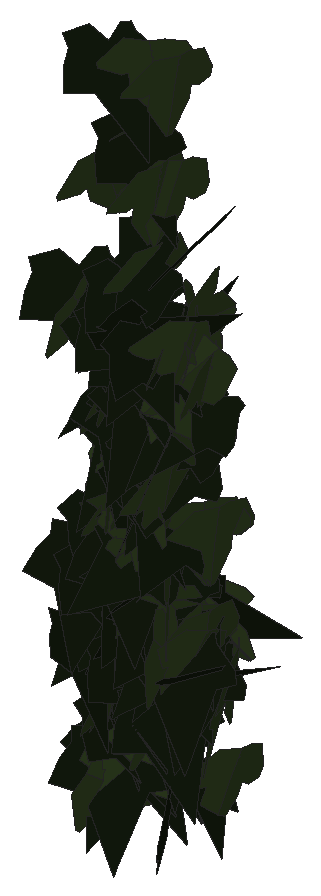
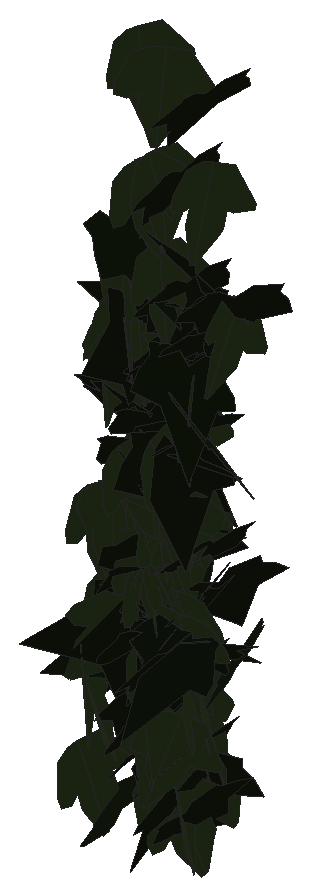
# SketchUp Ruby script. Lengths in inches.
U = 1.inch
M = Sketchup.active_model
def pt(a) = Geom::Point3d.new(a.map { |v| v * U })
def face(e, loops, mat)
  f = e.add_face(loops[0].map { |a| pt(a) })
  loops[1..].each { |l| e.add_face(l.map { |a| pt(a) }).erase! }
  f.material = f.back_material = mat if mat
  f
end
# faces: each face lists its corners as indices into pts; further lists are holes
def faces(e, pts, list, mat = nil) = list.each { |f| face(e, (f[0].is_a?(Array) ? f : [f]).map { |l| l.map { |i| pts[i] } }, mat) }
# xy, xz, yz: faces in a plane at the given z, y or x. An outline is a flat list of corners, or four numbers for a rectangle; further outlines are holes
def ring(l) = l.size == 4 ? [[l[0], l[1]], [l[2], l[1]], [l[2], l[3]], [l[0], l[3]]] : l.each_slice(2).to_a
def flat(e, list, mat, &to3) = list.each { |f| face(e, (f[0].is_a?(Array) ? f : [f]).map { |l| ring(l).map { |u, v| to3.(u, v) } }, mat) }
def xy(e, z, list, mat = nil) = flat(e, list, mat) { |x, y| [x, y, z] }
def xz(e, y, list, mat = nil) = flat(e, list, mat) { |x, z| [x, y, z] }
def yz(e, x, list, mat = nil) = flat(e, list, mat) { |y, z| [x, y, z] }
def lines(e, pts, list) = list.each { |a, b| e.add_line(pt(pts[a]), pt(pts[b])) }
# prism: a flat outline (further loops are holes) pulled along v
def prism(e, loops, v, mat = nil)
  f = face(e, loops, mat); d = Geom::Vector3d.new(v.map { |x| x * U })
  f.pushpull(f.normal.samedirection?(d) ? d.length : -d.length)
end
def box(e, o, s, mat = nil) = prism(e, [[o, [o[0] + s[0], o[1], o[2]], [o[0] + s[0], o[1] + s[1], o[2]], [o[0], o[1] + s[1], o[2]]]], [0, 0, s[2]], mat)
def at(x, y, z, deg = 0) = Geom::Transformation.translation(pt([x, y, z])) * Geom::Transformation.rotation(ORIGIN, Z_AXIS, deg.degrees)
def axes(o, x, y, z) = Geom::Transformation.new([*x, 0, *y, 0, *z, 0, *pt(o).to_a, 1])
def part(name) = M.definitions.add(name)
# library, detail: a bought-in or finely detailed component or shape, given as its bounding box
def library(name, o, s) = part(name).tap { |d| box(d.entities, o, s) }
def detail(e, o, s) = box(e.add_group.entities, o, s)
def put(e, d, t, mat = nil) = e.add_instance(d, t).tap { |i| i.material = mat if mat }
def group(e, t, mat = nil) = e.add_group.tap { |g| g.transformation = t; g.material = mat if mat }.entities
root = M.entities
M.materials.add("efeu1").color = [18, 25, 13]
M.materials.add("efeu2").color = [43, 57, 29]
c1 = part("ivyleaf_9")
p = [[1.54,2.16,1.25],[1.36,2.04,1.19],[-0.21,0.99,0.68],[-0.71,1.11,0.82],[-0.85,0.86,0.67],[-0.8,0.17,0.21],
  [-0.9,-0.01,0.1],[-0.67,-0.16,-0.02],[-0.08,-0.08,-0.05],[-0.03,-0.6,-0.4],[0.65,-0.88,-0.66],[0.83,-0.6,-0.49],
  [1.29,-0.42,-0.43],[1.8125,-0.07,-0.26],[1.21,0.44,0.15]]
faces(c1.entities,p,[[0,1,2,3,4,5,6,7,8,9,10,11,12,13,14]],"efeu1")
c2 = part("ivyleaf_10")
p = [[0,0.5,-0.03],[-0.0625,2.02,-0.43],[-0.19,2.01,-0.46],[-0.54,1.05,-0.29],[-0.52,0.625,-0.18],[-0.83,0.76,-0.28],
  [-1.16,0.64,-0.33],[-1.15,0.33,-0.24],[-0.77,-0.39,0.02],[-0.3,-0.51,0.16],[0.04,-0.48,0.23],[-0.02,2.01,-0.4375],
  [-0.06,2.01,-0.43],[0.04,-0.49,0.23],[0.67,-0.49,0.14],[1.38,0.36,-0.2],[1.375,0.51,-0.24],[0.81,0.65,-0.19],
  [0.62,0.59,-0.15],[0.6,1.09,-0.28],[0.5,1.23,-0.31]]
faces(c2.entities,p,[[0,1,2,3,4,5,6,7,8,9,10],[11,12,0,13,14,15,16,17,18,19,20]],"efeu2")
put(root,c1,axes([21.94,224.4,223.21],[-0.14106,-0.45838,0.14138],[-0.02129,-0.14124,-0.47916],[0.47922,-0.1412,0.02033]))
put(root,c2,axes([22,223.4,229.6875],[-0.04189,-0.41196,-0.28024],[0.08454,0.27127,-0.41142],[0.49102,-0.08185,0.04693]))
put(root,c1,axes([21.8,224.47,224.08],[0.14653,-0.46701,0.1021],[0.01791,-0.10136,-0.48929],[0.47771,0.14705,-0.01298]))
put(root,c1,axes([22.24,224.13,228.68],[-0.45749,0.18707,-0.07557],[0.06415,-0.04269,-0.49403],[-0.19128,-0.46172,0.01506]))
put(root,c1,axes([21.92,224.43,225.625],[0.47113,0.13259,-0.10227],[-0.11672,0.04106,-0.48445],[-0.12006,0.48035,0.06964]))
put(root,c1,axes([21.97,223.72,226.14],[-0.15755,-0.47379,-0.02647],[0.00905,0.02488,-0.4993],[0.47444,-0.15781,0.00073]))
put(root,c1,axes([22.13,224.22,225.4],[-0.40668,-0.28423,0.06183],[0.04349,-0.1645,-0.47016],[0.2876,-0.37703,0.15852]))
put(root,c1,axes([21.82,223.64,224.96],[0.20698,-0.44397,0.10024],[0.02843,-0.0973,-0.48962],[0.45426,0.20838,-0.01503]))
put(root,c2,axes([22.1,223.78,224.33],[0.19956,-0.45768,-0.02653],[-0.00921,0.02492,-0.49929],[0.45836,0.19976,0.00152]))
put(root,c1,axes([21.92,223.52,230.04],[-0.07806,-0.43601,-0.23195],[0.08242,0.22004,-0.44135],[0.48694,-0.10713,0.03752]))
put(root,c2,axes([22.03,224.38,223.27],[0.24348,-0.4249,0.10089],[0.09898,-0.05882,-0.48656],[0.42535,0.25691,0.05547]))
put(root,c1,axes([22.24,224.23,228.0625],[0.14218,0.45199,-0.15967],[-0.12515,-0.12577,-0.46746],[-0.46274,0.17289,0.07737]))
put(root,c2,axes([22.16,223.94,228.39],[0.03167,-0.48427,-0.12032],[0.01668,0.12152,-0.48472],[0.49872,0.02669,0.02385]))
put(root,c2,axes([22.0625,224.3,225.71],[0.49949,-0.02245,0.00148],[0.00193,0.01006,-0.49989],[0.02241,0.49939,0.01014]))
put(root,c2,axes([22.07,224.125,224.64],[0.15197,-0.43923,0.18435],[0.11422,-0.15426,-0.46169],[0.46245,0.18244,0.05346]))
put(root,c2,axes([22.11,224.28,226],[0.48816,-0.10408,-0.02949],[-0.02293,0.03365,-0.49834],[0.10572,0.48789,0.02808]))
put(root,c1,axes([22.3,223.95,229.1],[0.02989,0.49897,0.01184],[-0.04365,0.01443,-0.49788],[-0.49719,0.02873,0.04442]))
put(root,c2,axes([22.1,224.49,224.3],[-0.38098,-0.28174,-0.15963],[0.15804,0.05336,-0.47136],[0.28263,-0.40961,0.0484]))
put(root,c2,axes([22.24,223.84,228.71],[0.13184,-0.39925,-0.27058],[-0.02577,0.27428,-0.41726],[0.48162,0.12397,0.05174]))
put(root,c2,axes([22.22,223.62,231.625],[-0.16859,-0.4393,-0.1691],[0.05535,0.15987,-0.47051],[0.46745,-0.17737,-0.00527]))
put(root,c2,axes([22.3,224.15,223.08],[-0.17886,-0.4356,0.1681],[-0.02787,-0.16973,-0.46948],[0.46608,-0.17731,0.03644]))
put(root,c2,axes([22.27,223.71,227.36],[0.21185,-0.33164,-0.30844],[-0.03998,0.32549,-0.37743],[0.45113,0.18458,0.11139]))
put(root,c1,axes([21.98,223.89,226.74],[0.1924,-0.39818,-0.23331],[0.03433,0.26442,-0.42297],[0.46022,0.14674,0.12909]))
put(root,c1,axes([22.01,223.75,226.03],[0.1514,-0.44552,-0.16908],[0.00989,0.18031,-0.46625],[0.47643,0.13783,0.06341]))
put(root,c2,axes([21.99,224.19,227.0625],[0.22119,0.12942,-0.42933],[0.35634,0.23988,0.2559],[0.27221,-0.41918,0.01388]))
put(root,c2,axes([22.17,223.58,223.24],[-0.09658,-0.29582,-0.39136],[0.20151,0.33975,-0.30653],[0.44729,-0.21693,0.05359]))
put(root,c2,axes([22.31,223.9375,226.95],[-0.04002,-0.49587,-0.05012],[0.01628,0.04896,-0.49733],[0.49813,-0.04144,0.01223]))
put(root,c1,axes([22.11,224.41,223.4375],[0.19119,-0.40496,-0.22238],[-0.09078,0.20306,-0.4478],[0.453,0.2116,0.00412]))
put(root,c2,axes([22.28,224.14,227.43],[-0.30039,-0.36289,-0.16757],[0.11316,0.12383,-0.47102],[0.38336,-0.3209,0.00774]))
put(root,c1,axes([22.41,224.16,227.79],[-0.43365,-0.24817,-0.01892],[0.01559,0.01086,-0.49964],[0.2484,-0.43393,-0.00169]))
put(root,c1,axes([22.0625,224.04,223.94],[0.20297,-0.42801,-0.16004],[0.01982,0.18319,-0.46481],[0.45652,0.18234,0.09133]))
put(root,c1,axes([22.1,223.87,233.01],[0.07746,-0.47126,-0.14805],[0.04853,0.15639,-0.47243],[0.49157,0.05882,0.06997]))
put(root,c2,axes([22.42,224.32,224.26],[-0.08147,0.45907,0.18059],[-0.19019,0.13966,-0.44082],[-0.45518,-0.14052,0.15186]))
put(root,c1,axes([22.28,223.78,223.52],[-0.31289,-0.28954,-0.26128],[0.17901,0.19098,-0.42601],[0.34649,-0.36013,-0.01585]))
put(root,c2,axes([22.44,224.22,227.01],[-0.09457,-0.49093,-0.00649],[-0.01044,0.00862,-0.49982],[0.49086,-0.0944,-0.01188]))
put(root,c2,axes([22.46,224.28,223.41],[-0.11639,-0.41597,0.25184],[-0.02631,-0.25319,-0.43035],[0.48555,-0.11343,0.03705]))
put(root,c2,axes([22.4,224.375,228.03],[0.03222,-0.45959,0.19427],[0.0448,-0.19122,-0.45981],[0.49695,0.04703,0.02886]))
put(root,c1,axes([22.18,224.53,225.41],[0.13366,-0.46723,-0.11759],[0.02391,0.12832,-0.48266],[0.48121,0.1234,0.05664]))
put(root,c1,axes([22.28,224.08,225.65],[-0.03347,-0.39023,0.31081],[0.00482,-0.31175,-0.39088],[0.49886,-0.02317,0.02463]))
put(root,c1,axes([22.32,224.05,228.13],[-0.08308,-0.49088,0.04616],[0.00074,-0.04693,-0.49779],[0.49305,-0.08265,0.00853]))
put(root,c2,axes([22.48,224.1875,227.35],[0.12474,-0.46693,-0.12813],[-0.00721,0.13051,-0.48261],[0.48414,0.12225,0.02583]))
put(root,c2,axes([22.45,223.62,227.52],[-0.42062,0.25374,-0.09322],[0.04942,-0.09734,-0.48794],[-0.26577,-0.41969,0.0568]))
put(root,c2,axes([22.55,223.83,223.56],[0.43188,0.17249,-0.18364],[-0.1787,-0.0472,-0.46459],[-0.17761,0.46693,0.02088]))
put(root,c2,axes([22.5625,224.15,227.51],[-0.22902,-0.43192,0.10486],[0.0064,-0.12115,-0.48506],[0.44442,-0.22083,0.06102]))
put(root,c1,axes([22.25,224.09,225.66],[0.16539,-0.40897,0.23536],[0.08479,-0.21958,-0.44113],[0.46417,0.18583,-0.00328]))
put(root,c2,axes([22.58,224.03,227.18],[0.01172,-0.48646,-0.11496],[0.0003,0.115,-0.4866],[0.49986,0.01134,0.00299]))
put(root,c1,axes([22.375,224,231.87],[0.13258,-0.45106,-0.1702],[-0.01608,0.17229,-0.4691],[0.48183,0.12986,0.03118]))
put(root,c1,axes([22.36,223.87,224.82],[0.14201,-0.46515,-0.11607],[0.00764,0.12324,-0.48451],[0.47935,0.13584,0.04211]))
put(root,c1,axes([22.35,223.9,227.19],[0.30853,-0.38075,-0.09921],[-0.04041,0.09474,-0.48928],[0.39138,0.30993,0.02769]))
put(root,c2,axes([22.65,224.18,225.11],[-0.13041,-0.45343,0.16551],[0.0073,-0.17328,-0.46896],[0.48264,-0.11989,0.05182]))
put(root,c1,axes([22.77,223.9375,225.79],[-0.18876,0.29632,-0.35576],[0.0772,-0.35867,-0.33971],[-0.45652,-0.18317,0.08965]))
put(root,c1,axes([22.46,224.52,224.45],[-0.00589,-0.49996,0.00106],[0.0002,-0.00107,-0.5],[0.49997,-0.00589,0.00021]))
put(root,c2,axes([22.62,224.01,226.4],[-0.0325,-0.40155,0.29615],[0.0719,-0.29745,-0.39542],[0.49373,0.01689,0.07708]))
put(root,c2,axes([22.68,224.1,223.92],[-0.00281,-0.49354,0.08008],[-0.01114,-0.08,-0.49343],[0.49987,-0.00456,-0.01055]))
put(root,c2,axes([22.97,223.43,227.1],[0.12912,0.00471,-0.48302],[-0.46434,0.13899,-0.12277],[0.13311,0.48027,0.04027]))
put(root,c2,axes([22.76,224.08,226.42],[-0.35087,-0.33198,0.12916],[-0.0545,-0.12913,-0.47995],[0.35202,-0.35088,0.05443]))
put(root,c1,axes([22.4,224.25,223.92],[0.31325,-0.389,-0.02348],[-0.01964,0.01434,-0.49941],[0.38921,0.3138,-0.0063]))
put(root,c1,axes([22.6,224.12,229.25],[-0.19836,-0.43098,0.15783],[0.00535,-0.17409,-0.46868],[0.45894,-0.18425,0.07368]))
put(root,c2,axes([22.63,224.03,225.61],[0.19514,-0.45116,0.09154],[0.0579,-0.07459,-0.491],[0.45669,0.20223,0.02313]))
put(root,c1,axes([22.53,223.75,226.4375],[-0.12315,-0.46435,-0.13861],[0.04991,0.1301,-0.48019],[0.48202,-0.13211,0.01431]))
put(root,c2,axes([22.66,224.125,224.1],[0.32773,-0.3775,-0.00942],[-0.0076,0.00588,-0.49991],[0.37754,0.32781,-0.00188]))
put(root,c2,axes([22.68,223.875,224.97],[-0.00432,-0.40517,-0.29294],[0.04511,0.29144,-0.40377],[0.49794,-0.02992,0.03404]))
put(root,c1,axes([22.74,223.92,226.43],[-0.32491,-0.29571,0.23872],[-0.07447,-0.25845,-0.4215],[0.37268,-0.30945,0.12391]))
put(root,c1,axes([22.95,224.15,227.59],[-0.40349,0.29285,0.03787],[-0.02685,0.02748,-0.49852],[-0.29406,-0.40433,-0.00645]))
put(root,c2,axes([22.6875,224.02,226.13],[0.0068,-0.35343,0.35361],[0.08851,-0.3472,-0.34873],[0.49206,0.06734,0.05784]))
put(root,c1,axes([23.02,223.6875,230.44],[-0.48185,0.08509,0.10284],[-0.10463,-0.0016,-0.48893],[-0.08288,-0.4927,0.01934]))
put(root,c1,axes([22.6,224.34,225.44],[-0.10442,-0.46079,-0.1636],[0.03883,0.15895,-0.47247],[0.48743,-0.11137,0.00259]))
put(root,c1,axes([22.63,224.14,225.35],[-0.15736,-0.3763,0.2892],[0.03423,-0.31289,-0.3885],[0.47336,-0.10247,0.12424]))
put(root,c2,axes([22.77,224.02,227.73],[-0.37633,-0.3216,0.07032],[0.03687,-0.14731,-0.47638],[0.32713,-0.35337,0.13459]))
put(root,c2,axes([22.77,224.14,227.41],[0.06918,-0.49363,0.03931],[0.00198,-0.03942,-0.49844],[0.49519,0.06912,-0.0035]))
put(root,c2,axes([22.79,223.84,233.14],[-0.42334,-0.26551,-0.01687],[0.02375,-0.00614,-0.4994],[0.26498,-0.42363,0.01781]))
put(root,c1,axes([22.55,223.67,230.1],[0.08224,-0.44585,-0.21084],[0.00698,0.21478,-0.45147],[0.49314,0.07131,0.04155]))
put(root,c2,axes([22.8,223.85,230.38],[-0.11156,-0.48625,-0.03336],[0.00264,0.03362,-0.49886],[0.48739,-0.11148,-0.00493]))
put(root,c1,axes([22.5625,224.43,224.04],[0.06417,-0.48193,0.11673],[0.03763,-0.11264,-0.48569],[0.49444,0.07112,0.02181]))
put(root,c1,axes([22.75,224.09,228.4],[-0.31328,-0.38587,-0.05439],[0.06621,0.01606,-0.49534],[0.38402,-0.31756,0.04103]))
put(root,c2,axes([22.85,224.1,225.96],[-0.00777,-0.49854,-0.03738],[0.00574,0.0373,-0.49857],[0.49991,-0.00818,0.00514]))
put(root,c1,axes([22.63,223.8,229.26],[0.0193,-0.46495,-0.1829],[0.034,0.18384,-0.46373],[0.49847,0.00546,0.03871]))
put(root,c2,axes([22.89,224.41,227.77],[-0.06249,-0.48206,0.11708],[0.0013,-0.11817,-0.48583],[0.49608,-0.06042,0.01603]))
put(root,c1,axes([23.09,224.29,226.18],[-0.25021,-0.13658,0.41078],[-0.34266,-0.22745,-0.28434],[0.26453,-0.42381,0.02022]))
put(root,c2,axes([22.92,223.81,225.79],[-0.36661,-0.33997,0.0039],[-0.00307,-0.00242,-0.49998],[0.33998,-0.36663,-0.00031]))
put(root,c2,axes([22.98,223.83,225.62],[-0.31212,-0.37123,0.12151],[-0.05637,-0.1111,-0.48423],[0.38652,-0.31598,0.0275]))
put(root,c1,axes([22.87,223.85,228.4375],[-0.21058,-0.43759,0.11904],[-0.04803,-0.10899,-0.48561],[0.45094,-0.21595,0.00387]))
put(root,c1,axes([22.83,224.2,226.27],[-0.19202,-0.4608,-0.02815],[0.00408,0.0288,-0.49915],[0.46164,-0.19192,-0.0073]))
put(root,c1,axes([22.63,223.55,229.65],[-0.02207,-0.43396,-0.24737],[0.21056,0.21646,-0.39851],[0.45296,-0.12177,0.17319]))
put(root,c2,axes([22.95,223.7,231.58],[-0.08576,-0.49216,-0.02062],[0.00497,0.02006,-0.49957],[0.49256,-0.08589,0.00145]))
put(root,c2,axes([23.03,223.96,231.53],[-0.15897,-0.46181,0.10705],[-0.00468,-0.11138,-0.48741],[0.47403,-0.15597,0.03109]))
put(root,c2,axes([23.35,223.625,228.31],[-0.03833,-0.00846,0.49846],[-0.49776,-0.02703,-0.03874],[0.02761,-0.4992,-0.00635]))
put(root,c2,axes([23.12,224.23,225.45],[-0.31345,-0.36633,0.13248],[-0.0849,-0.10172,-0.48213],[0.38019,-0.32474,0.00156]))
put(root,c1,axes([23.01,223.79,227.91],[-0.2908,0.17144,-0.36884],[0.29429,-0.2243,-0.33628],[-0.28076,-0.41267,0.02955]))
put(root,c1,axes([23.12,224.18,225.3],[-0.39925,-0.28699,0.09073],[-0.00426,-0.14532,-0.4784],[0.30096,-0.38278,0.1136]))
put(root,c1,axes([23.14,224.14,225.52],[-0.47228,-0.10579,-0.12552],[0.12348,0.02297,-0.48397],[0.10817,-0.48814,0.00443]))
put(root,c1,axes([22.76,224.6875,223.13],[0.12463,-0.43072,0.22124],[0.13497,-0.18849,-0.44301],[0.46503,0.17014,0.06928]))
put(root,c1,axes([23.1,224,227.87],[-0.35823,-0.3486,-0.01234],[0.00864,0.00881,-0.49985],[0.34871,-0.35833,-0.00028]))
put(root,c2,axes([23.12,223.83,229.44],[0.12053,-0.46037,-0.1534],[-0.02356,0.15232,-0.47565],[0.48468,0.12189,0.01502]))
put(root,c1,axes([22.875,224,225.3125],[-0.06695,-0.38475,-0.31223],[0.13335,0.28945,-0.38527],[0.47722,-0.13485,0.06385]))
put(root,c1,axes([22.92,223.91,224.36],[-0.01717,-0.44769,-0.22198],[0.01521,0.22154,-0.44798],[0.49947,-0.02214,0.00601]))
put(root,c2,axes([23.01,223.97,226.1],[-0.10977,0.38906,-0.29425],[0.04997,-0.29105,-0.40348],[-0.48524,-0.11799,0.02502]))
put(root,c1,axes([23.16,223.96,229.19],[0.0294,0.18582,0.46326],[0.11212,0.44974,-0.18752],[-0.48638,0.11491,-0.01522]))
put(root,c1,axes([23.21,223.46,222.75],[0.04023,-0.02577,0.49771],[0.03226,0.49842,0.0232],[-0.49733,0.03025,0.04176]))
put(root,c1,axes([22.77,223.36,229.33],[0.13362,-0.0385,0.48027],[0.4734,0.10326,-0.12343],[-0.08968,0.4877,0.06404]))
put(root,c1,axes([23.03,223.33,229.73],[0.10058,-0.29104,-0.39393],[-0.13725,0.36929,-0.30788],[0.47015,0.17007,-0.0056]))
put(root,c1,axes([23.37,223.95,230.75],[-0.25805,0.40027,-0.1523],[0.01086,-0.17163,-0.46949],[-0.42813,-0.24561,0.07988]))
put(root,c2,axes([22.99,224.4,225.55],[-0.36777,-0.1714,-0.29217],[0.27481,0.10117,-0.40527],[0.19805,-0.45868,0.01979]))
put(root,c1,axes([22.81,224.36,225.48],[0.10184,0.1432,-0.4681],[0.26555,0.3855,0.1757],[0.41123,-0.2844,0.00246]))
put(root,c1,axes([23.01,223.88,226.91],[-0.09876,-0.40179,0.28074],[0.06607,-0.29468,-0.3985],[0.48568,-0.04162,0.11129]))
put(root,c2,axes([23.18,223.91,228.92],[-0.20459,-0.39467,0.22886],[0.05729,-0.27106,-0.41623],[0.45261,-0.14409,0.15613]))
put(root,c2,axes([23.25,223.53,227.67],[-0.05417,-0.497,-0.00741],[0.00051,0.0074,-0.49994],[0.49706,-0.05417,-0.00029]))
put(root,c2,axes([23.27,223.66,233.1875],[-0.17102,-0.4698,0.00626],[-0.0019,-0.00597,-0.49996],[0.46984,-0.17103,0.00026]))
put(root,c2,axes([23.35,223.86,229.72],[0.21883,-0.301,-0.33394],[-0.14671,0.30326,-0.36948],[0.42496,0.25969,0.04441]))
put(root,c2,axes([23.22,223.37,225.47],[0.14945,-0.35275,-0.3213],[0.06709,0.34888,-0.35183],[0.4724,0.06205,0.15161]))
put(root,c1,axes([23.52,224.02,228.36],[-0.49288,0.04411,0.07155],[-0.07549,-0.04512,-0.49221],[-0.03697,-0.496,0.05114]))
put(root,c1,axes([23.2,224.16,225.01],[-0.17744,-0.46578,-0.03958],[0.01209,0.03775,-0.49843],[0.4673,-0.17784,-0.00214]))
put(root,c2,axes([23.5,223.89,229.22],[-0.24142,-0.2385,0.3672],[-0.18947,-0.32112,-0.33314],[0.39474,-0.3,0.06467]))
put(root,c2,axes([23.4,223.91,229.64],[-0.00595,0.0968,0.4905],[-0.20592,0.44653,-0.09062],[-0.45559,-0.20309,0.03455]))
put(root,c2,axes([23.36,224.1,226.97],[-0.29389,-0.40432,-0.01254],[0.03501,-0.00998,-0.49867],[0.40299,-0.29399,0.03418]))
put(root,c2,axes([23.42,223.6875,229.59],[-0.20119,-0.43896,0.12976],[-0.0267,-0.13024,-0.482],[0.45696,-0.20088,0.02897]))
put(root,c1,axes([23.45,224.07,228.59],[-0.45825,-0.19993,0.00577],[0.05154,-0.13198,-0.4795],[0.19326,-0.43887,0.14157]))
put(root,c2,axes([23.45,223.85,225.35],[-0.08199,-0.46385,0.1677],[-0.03402,-0.16427,-0.47102],[0.49206,-0.08865,-0.00463]))
put(root,c2,axes([23.46,224.53,223.47],[-0.10315,-0.4779,0.10475],[-0.0183,-0.10321,-0.48889],[0.4889,-0.10469,0.0038]))
put(root,c2,axes([23.34,224.46,224.37],[0.2785,-0.38955,0.14382],[0.08461,-0.1163,-0.47887],[0.40654,0.29107,0.00114]))
put(root,c2,axes([23.48,224.17,226.93],[-0.18556,-0.46426,-0.00538],[0.00042,0.00563,-0.49997],[0.46429,-0.18555,-0.0017]))
put(root,c2,axes([23.43,224.55,224.83],[0.2203,-0.43348,-0.11648],[0.0041,0.13169,-0.48233],[0.44883,0.21156,0.06157]))
put(root,c1,axes([23.2,223.6,224.84],[0.39525,0.12162,0.28105],[0.16546,0.30131,-0.36309],[-0.25768,0.38003,0.19794]))
put(root,c2,axes([23.49,223.96,225.6],[-0.11267,-0.48689,-0.01562],[0.01145,0.01338,-0.49969],[0.48701,-0.11296,0.00814]))
put(root,c1,axes([23.3125,223.75,225.26],[-0.29134,-0.29012,-0.28453],[0.24767,0.15078,-0.40734],[0.32216,-0.37828,0.05585]))
put(root,c2,axes([23.49,224.01,229.11],[0.10674,-0.45358,-0.18129],[-0.01386,0.18268,-0.46523],[0.48828,0.10435,0.02642]))
